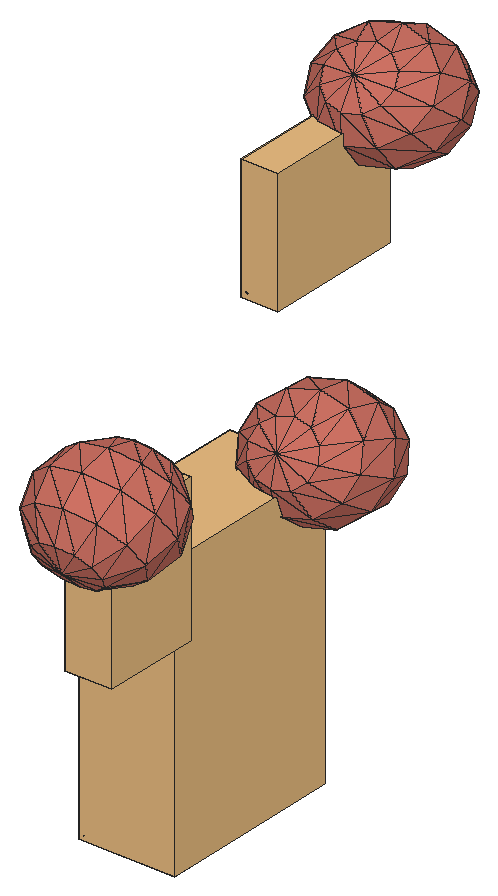
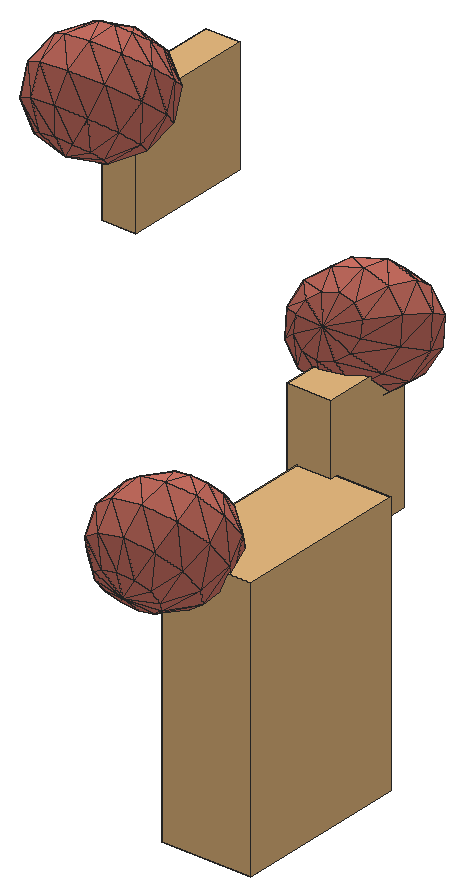
# SketchUp Ruby script. Lengths in inches.
U = 1.inch
M = Sketchup.active_model
def pt(a) = Geom::Point3d.new(a.map { |v| v * U })
def face(e, loops, mat)
  f = e.add_face(loops[0].map { |a| pt(a) })
  loops[1..].each { |l| e.add_face(l.map { |a| pt(a) }).erase! }
  f.material = f.back_material = mat if mat
  f
end
# faces: each face lists its corners as indices into pts; further lists are holes
def faces(e, pts, list, mat = nil) = list.each { |f| face(e, (f[0].is_a?(Array) ? f : [f]).map { |l| l.map { |i| pts[i] } }, mat) }
# xy, xz, yz: faces in a plane at the given z, y or x. An outline is a flat list of corners, or four numbers for a rectangle; further outlines are holes
def ring(l) = l.size == 4 ? [[l[0], l[1]], [l[2], l[1]], [l[2], l[3]], [l[0], l[3]]] : l.each_slice(2).to_a
def flat(e, list, mat, &to3) = list.each { |f| face(e, (f[0].is_a?(Array) ? f : [f]).map { |l| ring(l).map { |u, v| to3.(u, v) } }, mat) }
def xy(e, z, list, mat = nil) = flat(e, list, mat) { |x, y| [x, y, z] }
def xz(e, y, list, mat = nil) = flat(e, list, mat) { |x, z| [x, y, z] }
def yz(e, x, list, mat = nil) = flat(e, list, mat) { |y, z| [x, y, z] }
def lines(e, pts, list) = list.each { |a, b| e.add_line(pt(pts[a]), pt(pts[b])) }
# prism: a flat outline (further loops are holes) pulled along v
def prism(e, loops, v, mat = nil)
  f = face(e, loops, mat); d = Geom::Vector3d.new(v.map { |x| x * U })
  f.pushpull(f.normal.samedirection?(d) ? d.length : -d.length)
end
def box(e, o, s, mat = nil) = prism(e, [[o, [o[0] + s[0], o[1], o[2]], [o[0] + s[0], o[1] + s[1], o[2]], [o[0], o[1] + s[1], o[2]]]], [0, 0, s[2]], mat)
def at(x, y, z, deg = 0) = Geom::Transformation.translation(pt([x, y, z])) * Geom::Transformation.rotation(ORIGIN, Z_AXIS, deg.degrees)
def axes(o, x, y, z) = Geom::Transformation.new([*x, 0, *y, 0, *z, 0, *pt(o).to_a, 1])
def part(name) = M.definitions.add(name)
# library, detail: a bought-in or finely detailed component or shape, given as its bounding box
def library(name, o, s) = part(name).tap { |d| box(d.entities, o, s) }
def detail(e, o, s) = box(e.add_group.entities, o, s)
def put(e, d, t, mat = nil) = e.add_instance(d, t).tap { |i| i.material = mat if mat }
def group(e, t, mat = nil) = e.add_group.tap { |g| g.transformation = t; g.material = mat if mat }.entities
root = M.entities
M.materials.add("green").color = [174, 139, 102]
M.materials.add("vio").color = [206, 114, 100]
c1 = library("3DGeom~102_Defintion",[-331.46,-500,-168.38],[662.92,1000,336.76])
c2 = part("3DGeom~103_Defintion")
p = [[302.66,-500,-146.11],[317.99,-495.14,-154.33],[299.97,-497.07,-128.32],[317.99,-495.14,-154.33],[302.66,-500,-146.11],[309.56,-498.4,-152.34],
  [299.97,-497.07,-128.32],[317.99,-495.14,-154.33],[312.61,-489.29,-118.76],[312.61,-489.29,-118.76],[317.99,-495.14,-154.33],[327.95,-484.43,-126.98],
  [317.99,-495.14,-154.33],[325.71,-491.1,-151.56],[330.64,-487.36,-144.77],[327.95,-484.43,-126.98],[317.99,-495.14,-154.33],[330.64,-487.36,-144.77],
  [302.66,-500,-146.11],[299.97,-497.07,-128.32],[299.15,-499.51,-137.32],[327.95,-484.43,-126.98],[330.64,-487.36,-144.77],[331.46,-484.92,-135.77],
  [299.97,-497.07,-128.32],[312.61,-489.29,-118.76],[304.89,-493.33,-121.53],[312.61,-489.29,-118.76],[327.95,-484.43,-126.98],[321.05,-486.03,-120.75],
  [-317.36,495.99,133.65],[-331.46,484.07,150.24],[-328.26,482.74,159.03],[-317.36,495.99,133.65],[-328.26,482.74,159.03],[-321.59,483.72,165.67],
  [-317.36,495.99,133.65],[-321.59,483.72,165.67],[-313.24,486.75,168.38],[-317.36,495.99,133.65],[-330.32,487.36,141.66],[-331.46,484.07,150.24],
  [-317.36,495.99,133.65],[-313.24,486.75,168.38],[-305.4375,491.02,166.44],[-317.36,495.99,133.65],[-325.17,491.72,135.59],[-330.32,487.36,141.66],
  [-317.36,495.99,133.65],[-305.4375,491.02,166.44],[-300.28,495.38,160.37],[-317.36,495.99,133.65],[-300.28,495.38,160.37],[-299.15,498.67,151.79],
  [-317.36,495.99,133.65],[-299.15,498.67,151.79],[-302.34,500,143.01],[-317.36,495.99,133.65],[-302.34,500,143.01],[-309.01,499.02,136.36]]
faces(c2.entities,p,[[0,1,2],[3,4,5],[6,7,8],[9,10,11],[12,13,14],[15,16,17],[18,19,20],[21,22,23],
  [24,25,26],[27,28,29],[30,31,32],[33,34,35],[36,37,38],[39,40,41],[42,43,44],[45,46,47],
  [48,49,50],[51,52,53],[54,55,56],[57,58,59]],"green")
c3 = library("3DGeom~104_Defintion",[-334.52,-500,-160.51],[669.04,1000,321.02])
c4 = part("3DGeom~105_Defintion")
p = [[-306.36,-487.18,-90.84],[-301.3,-484.5,-160.51],[-278.52,-498.77,-106.98],[-278.52,-498.77,-106.98],[-301.3,-484.5,-160.51],[-275.99,-497.43,-141.8125],
  [-301.3,-484.5,-160.51],[-286.29,-491.76,-155.1],[-275.99,-497.43,-141.8125],[-331.67,-474.24,-109.53],[-301.3,-484.5,-160.51],[-306.36,-487.18,-90.84],
  [-329.14,-472.9,-144.36],[-301.3,-484.5,-160.51],[-331.67,-474.24,-109.53],[-301.3,-484.5,-160.51],[-329.14,-472.9,-144.36],[-316.98,-477.6,-156.58],
  [-329.14,-472.9,-144.36],[-331.67,-474.24,-109.53],[-334.52,-471.68,-127.14],[-278.52,-498.77,-106.98],[-275.99,-497.43,-141.8125],[-273.14,-500,-124.2],
  [-331.67,-474.24,-109.53],[-306.36,-487.18,-90.84],[-321.37,-479.92,-96.24],[-306.36,-487.18,-90.84],[-278.52,-498.77,-106.98],[-290.68,-494.08,-94.77],
  [313.125,494.74,102.45],[292.39,466.72,160.51],[309.13,461.51,157.36],[313.125,494.74,102.45],[309.13,461.51,157.36],[324.16,461.46,147.27],
  [313.125,494.74,102.45],[324.16,461.46,147.27],[333.45,466.57,132.95],[313.125,494.74,102.45],[333.45,466.57,132.95],[334.52,475.47,118.24],
  [313.125,494.74,102.45],[278.4375,475.68,155.88],[292.39,466.72,160.51],[313.125,494.74,102.45],[334.52,475.47,118.24],[327.08,485.78,107.08],
  [313.125,494.74,102.45],[271,485.99,144.72],[278.4375,475.68,155.88],[313.125,494.74,102.45],[272.07,494.89,130.01],[271,485.99,144.72],
  [313.125,494.74,102.45],[281.36,500,115.69],[272.07,494.89,130.01],[313.125,494.74,102.45],[296.39,499.94,105.61],[281.36,500,115.69]]
faces(c4.entities,p,[[0,1,2],[3,4,5],[6,7,8],[9,10,11],[12,13,14],[15,16,17],[18,19,20],[21,22,23],
  [24,25,26],[27,28,29],[30,31,32],[33,34,35],[36,37,38],[39,40,41],[42,43,44],[45,46,47],
  [48,49,50],[51,52,53],[54,55,56],[57,58,59]],"green")
c5 = part("3DGeom~222_Defintion")
p = [[138.17,-187.6,-427.375],[-199.9375,-99.75,-443.62],[24.02,0,-500],[340.4,-62.72,-359.51],[-304.37,62.72,-390.49],[340.4,-62.72,-359.51],
  [241.54,99.75,-422.41],[-96.57,187.6,-438.65],[-101.08,-262.21,-380.72],[-370.32,-172.76,-268.37],[-430.61,-78.97,-237.69],[-430.61,-78.97,-237.69],
  [-386.39,181.65,-235.57],[137.11,262.21,-369.28],[-386.39,181.65,-235.57],[-191.28,324.93,-259.77],[137.11,262.21,-369.28],[-191.28,324.93,-259.77],
  [215.3,-324.93,-240.23],[407.19,-181.65,-197.45],[407.19,-181.65,-197.45],[340.4,-62.72,-359.51],[451.41,78.97,-195.32],[340.4,-62.72,-359.51],
  [241.54,99.75,-422.41],[241.54,99.75,-422.41],[394.34,172.77,-231.63],[394.34,172.77,-231.63],[137.11,262.21,-369.28],[-304.37,62.72,-390.49],
  [-430.61,-78.97,-237.69],[-477.97,-10.3,-148.25],[-304.37,62.72,-390.49],[-386.39,181.65,-235.57],[-34.29,-381.14,-218.65],[-313.24,-266.5625,-232.06],
  [-101.08,-262.21,-380.72],[-34.29,-381.14,-218.65],[-313.24,-266.5625,-232.06],[394.34,172.77,-231.63],[137.11,262.21,-369.28],[334.05,266.5625,-200.96],
  [137.11,262.21,-369.28],[-191.28,324.93,-259.77],[55.09,381.14,-214.36],[334.05,266.5625,-200.96],[137.11,262.21,-369.28],[55.09,381.14,-214.36],
  [489.98,10.3,-101.75],[407.19,-181.65,-197.45],[-370.32,-172.76,-268.37],[-313.24,-266.5625,-232.06],[-441.48,-199.49,-21.21],[-370.32,-172.76,-268.37],
  [-191.28,324.93,-259.77],[-424.03,225.18,-20.37],[-191.28,324.93,-259.77],[-234.74,375.19,-11.28],[-191.28,324.93,-259.77],[-234.74,375.19,-11.28],
  [234.74,-375.19,11.28],[-34.29,-381.14,-218.65],[215.3,-324.93,-240.23],[424.03,-225.18,20.37],[234.74,-375.19,11.28],[215.3,-324.93,-240.23],
  [215.3,-324.93,-240.23],[-499.7,14.83,-24.01],[-34.29,-381.14,-218.65],[-274.68,-335.23,-138.48],[-313.24,-266.5625,-232.06],[-313.24,-266.5625,-232.06],
  [-274.68,-335.23,-138.48],[441.48,199.49,21.21],[334.05,266.5625,-200.96],[-17.45,-424.67,-0.84],[-34.29,-381.14,-218.65],[234.74,-375.19,11.28],
  [-34.29,-381.14,-218.65],[334.05,266.5625,-200.96],[286.69,335.23,-111.52],[286.69,335.23,-111.52],[17.45,424.67,0.84],[286.69,335.23,-111.52],
  [499.7,-14.83,24.01],[-264.96,-360.36,-12.73],[-274.68,-335.23,-138.48],[-264.96,-360.36,-12.73],[264.96,360.36,12.73],[286.69,335.23,-111.52],
  [264.96,360.36,12.73],[-489.98,-10.3,101.75],[-264.96,-360.36,-12.73],[-286.69,-335.23,111.52],[-286.69,-335.23,111.52],[-334.05,-266.5625,200.96],
  [-334.05,-266.5625,200.96],[-394.34,-172.77,231.63],[-451.41,-78.97,195.32],[-394.34,-172.77,231.63],[-407.19,181.65,197.45],[-234.74,375.19,-11.28],
  [-407.19,181.65,197.45],[-55.09,-381.14,214.36],[-286.69,-335.23,111.52],[-234.74,375.19,-11.28],[-407.19,181.65,197.45],[-215.3,324.93,240.23],
  [-215.3,324.93,240.23],[191.28,-324.93,259.77],[191.28,-324.93,259.77],[234.74,-375.19,11.28],[-215.3,324.93,240.23],[34.29,381.14,218.65],
  [264.96,360.36,12.73],[386.39,-181.65,235.57],[191.28,-324.93,259.77],[274.68,335.23,138.48],[264.96,360.36,12.73],[274.68,335.23,138.48],
  [477.97,10.3,148.25],[430.61,78.97,237.69],[370.32,172.77,268.37],[313.24,266.5625,232.06],[-407.19,181.65,197.45],[-137.11,-262.21,369.28],
  [-137.11,-262.21,369.28],[-334.05,-266.5625,200.96],[274.68,335.23,138.48],[101.08,262.21,380.72],[274.68,335.23,138.48],[101.08,262.21,380.72],
  [313.24,266.5625,232.06],[-340.4,62.72,359.51],[-394.34,-172.77,231.63],[-407.19,181.65,197.45],[-340.4,62.72,359.51],[-215.3,324.93,240.23],
  [-407.19,181.65,197.45],[-340.4,62.72,359.51],[-241.54,-99.75,422.41],[-394.34,-172.77,231.63],[-334.05,-266.5625,200.96],[-334.05,-266.5625,200.96],
  [-137.11,-262.21,369.28],[96.57,-187.6,438.65],[-55.09,-381.14,214.36],[-55.09,-381.14,214.36],[191.28,-324.93,259.77],[34.29,381.14,218.65],
  [-138.17,187.6,427.375],[34.29,381.14,218.65],[101.08,262.21,380.72],[-340.4,62.72,359.51],[-394.34,-172.77,231.63],[-241.54,-99.75,422.41],
  [313.24,266.5625,232.06],[199.9375,99.75,443.62],[313.24,266.5625,232.06],[370.32,172.77,268.37],[304.37,-62.72,390.49],[191.28,-324.93,259.77],
  [386.39,-181.65,235.57],[304.37,-62.72,390.49],[370.32,172.77,268.37],[304.37,-62.72,390.49],[430.61,78.97,237.69],[304.37,-62.72,390.49],
  [191.28,-324.93,259.77],[370.32,172.77,268.37],[304.37,-62.72,390.49],[-24.02,0,500],[304.37,-62.72,390.49]]
faces(c5.entities,p,[[0,1,2],[3,0,2],[2,1,4],[5,2,6],[2,4,7],[6,2,7],[8,9,1],[0,8,1],
  [1,9,10],[1,11,4],[7,4,12],[6,7,13],[7,14,15],[16,7,17],[18,8,0],[19,18,0],
  [20,0,21],[22,23,24],[22,25,26],[27,6,28],[29,30,31],[32,31,33],[34,35,36],[18,37,8],
  [8,38,9],[39,40,41],[42,43,44],[45,46,47],[48,49,23],[48,23,22],[50,51,52],[30,53,52],
  [54,33,55],[56,55,57],[47,58,59],[60,61,62],[63,64,65],[63,66,49],[31,30,52],[33,31,67],
  [33,67,55],[68,69,70],[71,72,52],[22,26,73],[26,74,73],[75,69,76],[77,75,78],[79,47,80],
  [81,47,82],[47,59,82],[74,83,73],[84,63,49],[84,49,48],[48,22,73],[67,31,52],[75,85,69],
  [86,87,52],[83,88,73],[89,82,90],[84,48,73],[91,67,52],[55,67,91],[92,93,52],[94,95,52],
  [96,97,52],[98,91,52],[99,98,52],[55,91,100],[101,55,102],[103,85,75],[103,104,85],[105,106,107],
  [82,59,108],[109,103,75],[110,75,111],[82,112,113],[114,82,113],[115,116,64],[115,64,63],[88,117,73],
  [118,113,119],[120,115,63],[120,63,84],[120,84,73],[121,120,73],[122,121,73],[123,122,73],[117,123,73],
  [124,91,98],[125,104,103],[126,127,104],[128,113,129],[130,131,132],[121,115,120],[133,98,134],[135,98,136],
  [137,138,139],[140,141,142],[140,143,144],[145,144,146],[145,147,148],[149,137,150],[151,150,152],[153,154,155],
  [156,152,157],[158,157,159],[160,161,162],[121,163,115],[164,165,166],[137,139,150],[167,145,168],[169,157,170],
  [150,139,140],[171,140,144],[171,144,145],[152,150,171],[152,171,157],[157,145,172],[150,140,171],[157,171,145]],"vio")
c6 = part("3DGeom~223_Defintion")
p = [[134.41,-263.08,-369.41],[-98.49,-186.72,-438.75],[24.02,0,-500],[240.51,-101.38,-422.46],[-198.9,101.38,-443.57],[240.51,-101.38,-422.46],
  [140.09,186.72,-427.28],[-98.38,263.08,-380.59],[-305,-60.32,-390.52],[-368.53,175.6,-268.28],[-310.49,268.95,-231.92],[-310.49,268.95,-231.92],
  [51.17,-381.46,-214.55],[-194.61,-323.41,-259.93],[51.17,-381.46,-214.55],[240.51,-101.38,-422.46],[341.03,60.32,-359.48],[341.03,60.32,-359.48],
  [218.625,323.41,-240.08],[-30.37,381.46,-218.47],[-30.37,381.46,-218.47],[218.625,323.41,-240.08],[331.3,-268.95,-201.09],[240.51,-101.38,-422.46],
  [331.3,-268.95,-201.09],[240.51,-101.38,-422.46],[392.55,-175.6,-231.72],[392.55,-175.6,-231.72],[240.51,-101.38,-422.46],[341.03,60.32,-359.48],
  [-388.24,-178.7,-235.66],[-388.24,-178.7,-235.66],[-429.78,82.24,-237.65],[-305,-60.32,-390.52],[-429.78,82.24,-237.65],[-98.38,263.08,-380.59],
  [-310.49,268.95,-231.92],[-271.23,337.3,-138.32],[-98.38,263.08,-380.59],[-30.37,381.46,-218.47],[283.24,-337.3,-111.68],[51.17,-381.46,-214.55],
  [134.41,-263.08,-369.41],[283.24,-337.3,-111.68],[134.41,-263.08,-369.41],[331.3,-268.95,-201.09],[450.59,-82.24,-195.36],[409.04,178.7,-197.36],
  [341.03,60.32,-359.48],[218.625,323.41,-240.08],[409.04,178.7,-197.36],[-368.53,175.6,-268.28],[-429.78,82.24,-237.65],[-439.41,202.76,-21.11],
  [-310.49,268.95,-231.92],[-368.53,175.6,-268.28],[13.09,-424.78,0.63],[-238.58,-373.4375,-11.46],[-194.61,-323.41,-259.93],[-194.61,-323.41,-259.93],
  [-238.58,-373.4375,-11.46],[-388.24,-178.7,-235.66],[-194.61,-323.41,-259.93],[218.625,323.41,-240.08],[238.58,373.4375,11.46],[218.625,323.41,-240.08],
  [-13.09,424.78,-0.63],[218.625,323.41,-240.08],[238.58,373.4375,11.46],[-388.24,-178.7,-235.66],[-477.84,13.89,-148.24],[-429.78,82.24,-237.65],
  [-429.78,82.24,-237.65],[-238.58,-373.4375,-11.46],[-426.32,-222.03,-20.48],[-388.24,-178.7,-235.66],[-388.24,-178.7,-235.66],[-271.23,337.3,-138.32],
  [-310.49,268.95,-231.92],[331.3,-268.95,-201.09],[439.41,-202.76,21.11],[-261.25,362.3125,-12.55],[261.25,-362.3125,12.55],[261.25,-362.3125,12.55],
  [283.24,-337.3,-111.68],[283.24,-337.3,-111.68],[489.85,-13.89,-101.76],[426.32,222.03,20.48],[-499.83,-11.125,-24.01],[-261.25,362.3125,-12.55],
  [-271.23,337.3,-138.32],[261.25,-362.3125,12.55],[499.83,11.125,24.01],[-409.04,-178.7,197.36],[-489.85,13.89,101.76],[-450.59,82.24,195.36],
  [-392.55,175.6,231.72],[-331.3,268.95,201.09],[-331.3,268.95,201.09],[-283.24,337.3,111.68],[-283.24,337.3,111.68],[-261.25,362.3125,-12.55],
  [-218.625,-323.41,240.08],[-238.58,-373.4375,-11.46],[-218.625,-323.41,240.08],[-283.24,337.3,111.68],[30.37,-381.46,218.47],[-218.625,-323.41,240.08],
  [-51.17,381.46,214.55],[238.58,373.4375,11.46],[-51.17,381.46,214.55],[271.23,-337.3,138.32],[271.23,-337.3,138.32],[261.25,-362.3125,12.55],
  [194.61,323.41,259.93],[238.58,373.4375,11.46],[-51.17,381.46,214.55],[194.61,323.41,259.93],[271.23,-337.3,138.32],[388.24,178.7,235.66],
  [194.61,323.41,259.93],[310.49,-268.95,231.92],[368.53,-175.6,268.28],[429.78,-82.24,237.65],[477.84,-13.89,148.24],[-341.03,-60.32,359.48],
  [-341.03,-60.32,359.48],[-51.17,381.46,214.55],[-331.3,268.95,201.09],[310.49,-268.95,231.92],[271.23,-337.3,138.32],[305,60.32,390.52],
  [305,60.32,390.52],[-240.51,101.38,422.46],[-341.03,-60.32,359.48],[-240.51,101.38,422.46],[-140.09,-186.72,427.28],[-409.04,-178.7,197.36],
  [-218.625,-323.41,240.08],[-341.03,-60.32,359.48],[-409.04,-178.7,197.36],[-134.41,263.08,369.41],[-331.3,268.95,201.09],[-392.55,175.6,231.72],
  [-51.17,381.46,214.55],[-331.3,268.95,201.09],[-134.41,263.08,369.41],[194.61,323.41,259.93],[-51.17,381.46,214.55],[98.38,-263.08,380.59],
  [-218.625,-323.41,240.08],[30.37,-381.46,218.47],[310.49,-268.95,231.92],[98.38,-263.08,380.59],[-392.55,175.6,231.72],[-240.51,101.38,422.46],
  [368.53,-175.6,268.28],[98.38,-263.08,380.59],[310.49,-268.95,231.92],[388.24,178.7,235.66],[98.49,186.72,438.74],[305,60.32,390.52],
  [388.24,178.7,235.66],[429.78,-82.24,237.65],[198.9,-101.38,443.57],[368.53,-175.6,268.28],[429.78,-82.24,237.65],[98.38,-263.08,380.59],
  [-218.625,-323.41,240.08],[368.53,-175.6,268.28],[98.38,-263.08,380.59],[-24.02,0,500],[98.38,-263.08,380.59]]
faces(c6.entities,p,[[0,1,2],[0,2,3],[1,4,2],[5,2,6],[2,4,7],[2,7,6],[1,8,4],[8,9,4],
  [4,9,10],[4,11,7],[12,13,1],[14,1,0],[13,8,1],[15,6,16],[17,6,18],[6,7,19],
  [6,20,21],[22,0,23],[24,25,26],[27,28,29],[13,30,8],[31,32,33],[8,34,9],[35,36,37],
  [38,37,39],[40,41,42],[43,44,45],[27,29,46],[46,29,47],[48,49,50],[51,52,53],[54,55,53],
  [56,57,58],[56,59,41],[60,61,62],[47,63,64],[65,39,66],[67,66,68],[69,70,71],[72,70,53],
  [73,74,75],[74,70,76],[77,78,53],[79,27,80],[27,46,80],[39,37,81],[39,81,66],[82,56,41],
  [83,41,84],[85,79,80],[46,47,86],[86,47,87],[47,64,87],[46,86,80],[74,88,70],[70,88,53],
  [89,90,53],[91,85,80],[86,92,80],[86,87,92],[93,88,74],[93,94,88],[88,94,53],[94,95,53],
  [95,96,53],[96,97,53],[98,99,53],[100,101,53],[102,74,103],[104,93,74],[66,81,105],[106,57,56],
  [106,107,57],[66,105,108],[109,66,110],[111,106,56],[112,56,113],[87,64,114],[115,116,117],[118,91,80],
  [92,87,119],[87,120,119],[121,118,80],[122,121,80],[123,122,80],[124,123,80],[92,124,80],[92,119,124],
  [125,94,93],[126,95,94],[127,105,128],[129,106,130],[124,131,123],[124,119,132],[133,95,134],[135,96,95],
  [136,137,138],[136,139,140],[141,142,143],[144,145,146],[147,148,141],[149,150,151],[152,153,106],[141,154,155],
  [156,157,158],[159,160,161],[162,147,160],[163,164,165],[166,161,164],[167,136,168],[147,141,160],[169,164,170],
  [171,139,136],[171,155,139],[160,141,155],[164,136,172],[161,171,164],[161,160,171],[160,155,171],[164,171,136]],"vio")
c7 = library("3DGeom~100_Defintion",[-500,-440.78,-130.77],[1000,881.57,261.54])
c8 = part("3DGeom~101_Defintion")
p = [[450.26,-438.5,-76.98],[473.93,-418.23,-130.77],[473.01,-420.54,-57.59],[450.72,-437.34,-113.57],[473.93,-418.23,-130.77],[450.26,-438.5,-76.98],
  [473.93,-418.23,-130.77],[450.72,-437.34,-113.57],[460.6,-429.08,-126.5],[473.01,-420.54,-57.59],[473.93,-418.23,-130.77],[496.21,-401.44,-74.78],
  [473.93,-418.23,-130.77],[487.14,-407.6875,-125.23],[496.68,-400.28,-111.37],[473.93,-418.23,-130.77],[496.68,-400.28,-111.37],[450.72,-437.34,-113.57],
  [450.26,-438.5,-76.98],[446.9375,-440.78,-95.45],[496.68,-400.28,-111.37],[500,-397.99,-92.9],[450.26,-438.5,-76.98],[473.01,-420.54,-57.59],
  [459.8,-431.09,-63.125],[473.01,-420.54,-57.59],[486.33,-409.69,-61.85],[-483.04,428.3125,67.76],[-497.53,394.8,97.99],[-487.96,391.61,113.91],
  [-483.04,428.3125,67.76],[-487.96,391.61,113.91],[-473.84,395.01,125.91],[-483.04,428.3125,67.76],[-500,403.73,82.41],[-497.53,394.8,97.99],
  [-483.04,428.3125,67.76],[-473.84,395.01,125.91],[-458.96,404.09,130.77],[-483.04,428.3125,67.76],[-494.7,415.99,71.34],[-483.04,428.3125,67.76],
  [-458.96,404.09,130.77],[-447.31,416.41,127.18],[-483.04,428.3125,67.76],[-447.31,416.41,127.18],[-442,428.67,116.12],[-483.04,428.3125,67.76],
  [-444.47,437.6,100.54],[-454.05,440.79,84.62],[-483.04,428.3125,67.76],[-454.05,440.79,84.62],[-468.16,437.39,72.62],[-483.04,428.3125,67.76],
  [-442,428.67,116.12],[-444.47,437.6,100.54]]
faces(c8.entities,p,[[0,1,2],[3,4,5],[6,7,8],[9,10,11],[12,13,14],[11,15,16],[17,18,19],[11,20,21],
  [22,23,24],[25,11,26],[27,28,29],[30,31,32],[33,34,35],[36,37,38],[39,40,34],[41,42,43],
  [44,45,46],[47,48,49],[50,51,52],[53,54,55]],"green")
c9 = part("3DGeom~221_Defintion")
p = [[192.89,-154.12,-424.75],[-160.54,-146.25,-441.73],[24.02,0,-500],[348.39,12.78,-359.13],[-312.36,-12.78,-390.87],[-151.29,154.12,-441.28],
  [202.15,146.25,-424.3],[348.39,12.78,-359.13],[-14.3,-279.72,-376.55],[-302.09,-253.31,-265.09],[-389.74,-176.26,-235.73],[-389.74,-176.26,-235.73],
  [-429.08,84.92,-237.62],[-429.08,84.92,-237.62],[-286.06,266.94,-264.32],[50.33,279.72,-373.45],[50.33,279.72,-373.45],[-286.06,266.94,-264.32],
  [310.08,-266.94,-235.68],[449.88,-84.92,-195.39],[310.08,-266.94,-235.68],[192.89,-154.12,-424.75],[192.89,-154.12,-424.75],[348.39,12.78,-359.13],
  [410.54,176.26,-197.28],[202.15,146.25,-424.3],[326.11,253.31,-234.91],[50.33,279.72,-373.45],[202.15,146.25,-424.3],[326.11,253.31,-234.91],
  [-312.36,-12.78,-390.87],[-389.74,-176.26,-235.73],[-457.125,-119.85,-147.25],[-312.36,-12.78,-390.87],[-429.08,84.92,-237.62],[87.19,-377.43,-212.82],
  [-217.65,-330.375,-227.46],[-14.3,-279.72,-376.55],[310.08,-266.94,-235.68],[87.19,-377.43,-212.82],[-217.65,-330.375,-227.46],[326.11,253.31,-234.91],
  [50.33,279.72,-373.45],[238.45,330.375,-205.55],[50.33,279.72,-373.45],[-286.06,266.94,-264.32],[-66.39,377.43,-220.19],[238.45,330.375,-205.55],
  [50.33,279.72,-373.45],[-66.39,377.43,-220.19],[469.14,119.85,-102.75],[-302.09,-253.31,-265.09],[-217.65,-330.375,-227.46],[-362.6875,-292.5,-17.42],
  [-302.09,-253.31,-265.09],[-362.6875,-292.5,-17.42],[-286.06,266.94,-264.32],[-479.41,120.6875,-23.03],[-286.06,266.94,-264.32],[-344.18,308.23,-16.53],
  [-286.06,266.94,-264.32],[-344.18,308.23,-16.53],[-486.1875,-99.2,-23.36],[344.18,-308.23,16.53],[87.19,-377.43,-212.82],[310.08,-266.94,-235.68],
  [479.41,-120.6875,23.03],[344.18,-308.23,16.53],[-362.6875,-292.5,-17.42],[362.6875,292.5,17.42],[238.45,330.375,-205.55],[-217.65,-330.375,-227.46],
  [-159.06,-386.79,-132.93],[-362.6875,-292.5,-17.42],[87.19,-377.43,-212.82],[-217.65,-330.375,-227.46],[-116.72,413.19,-5.61],[171.07,386.79,-117.07],
  [116.72,-413.19,5.61],[87.19,-377.43,-212.82],[344.18,-308.23,16.53],[87.19,-377.43,-212.82],[362.6875,292.5,17.42],[486.1875,99.2,23.36],
  [-362.6875,-292.5,-17.42],[-142.01,-407.43,-6.82],[142.01,407.43,6.82],[362.6875,292.5,17.42],[-469.14,-119.85,102.75],[-362.6875,-292.5,-17.42],
  [-449.88,84.92,195.39],[-344.18,308.23,-16.53],[-171.07,-386.79,117.07],[-238.45,-330.375,205.55],[-238.45,-330.375,205.55],[-326.11,-253.31,234.91],
  [-362.6875,-292.5,-17.42],[-410.54,-176.26,197.28],[-362.6875,-292.5,-17.42],[-326.11,-253.31,234.91],[-362.6875,-292.5,-17.42],[-344.18,308.23,-16.53],
  [-310.08,266.94,235.68],[-310.08,266.94,235.68],[66.39,-377.43,220.2],[-310.08,266.94,235.68],[-87.19,377.43,212.82],[286.06,-266.94,264.32],
  [286.06,-266.94,264.32],[344.18,-308.23,16.53],[159.06,386.79,132.93],[362.6875,292.5,17.42],[429.08,-84.92,237.62],[286.06,-266.94,264.32],
  [457.125,119.85,147.25],[389.74,176.26,235.73],[302.09,253.31,265.09],[217.65,330.375,227.46],[217.65,330.375,227.46],[362.6875,292.5,17.42],
  [-50.33,-279.72,373.45],[-50.33,-279.72,373.45],[14.3,279.72,376.55],[14.3,279.72,376.55],[217.65,330.375,227.46],[-348.39,-12.78,359.13],
  [-310.08,266.94,235.68],[-348.39,-12.78,359.13],[-348.39,-12.78,359.13],[-326.11,-253.31,234.91],[-202.15,-146.25,424.3],[-326.11,-253.31,234.91],
  [-238.45,-330.375,205.55],[-238.45,-330.375,205.55],[-50.33,-279.72,373.45],[-87.19,377.43,212.82],[-310.08,266.94,235.68],[-192.89,154.12,424.75],
  [-87.19,377.43,212.82],[14.3,279.72,376.55],[151.29,-154.12,441.28],[66.39,-377.43,220.2],[66.39,-377.43,220.2],[286.06,-266.94,264.32],
  [217.65,330.375,227.46],[160.54,146.25,441.73],[217.65,330.375,227.46],[302.09,253.31,265.09],[-348.39,-12.78,359.13],[-326.11,-253.31,234.91],
  [-202.15,-146.25,424.3],[312.36,12.78,390.87],[-310.08,266.94,235.68],[-348.39,-12.78,359.13],[-192.89,154.12,424.75],[302.09,253.31,265.09],
  [312.36,12.78,390.87],[389.74,176.26,235.73],[312.36,12.78,390.87],[286.06,-266.94,264.32],[429.08,-84.92,237.62],[312.36,12.78,390.87],
  [286.06,-266.94,264.32],[302.09,253.31,265.09],[312.36,12.78,390.87],[-348.39,-12.78,359.13],[-24.02,0,500],[312.36,12.78,390.87]]
faces(c9.entities,p,[[0,1,2],[3,0,2],[2,1,4],[2,4,5],[6,2,5],[7,2,6],[8,9,1],[0,8,1],
  [1,9,10],[1,11,4],[5,4,12],[5,13,14],[6,5,15],[16,5,17],[18,8,0],[19,20,21],
  [19,22,23],[24,23,25],[26,6,27],[24,28,29],[30,31,32],[33,32,34],[35,36,37],[38,39,8],
  [8,40,9],[41,42,43],[44,45,46],[47,48,49],[50,19,23],[50,23,24],[51,52,53],[31,54,55],
  [56,34,57],[58,57,59],[49,60,61],[34,32,62],[34,62,57],[63,64,65],[66,67,20],[32,31,68],
  [66,20,19],[24,29,69],[29,70,69],[71,72,73],[74,72,75],[49,61,76],[47,49,77],[77,49,76],
  [78,72,79],[80,78,81],[47,77,82],[50,24,69],[83,66,19],[83,19,50],[62,32,84],[78,85,72],
  [72,85,73],[77,86,87],[77,76,86],[83,50,69],[88,62,89],[57,62,88],[57,88,90],[91,57,90],
  [85,92,73],[92,93,73],[94,95,96],[97,88,98],[99,97,100],[101,90,102],[76,61,103],[104,85,78],
  [104,92,85],[76,105,106],[86,76,106],[107,104,78],[108,78,109],[86,110,111],[86,106,110],[112,113,67],
  [112,67,66],[114,83,69],[115,114,69],[116,115,69],[117,116,69],[110,118,119],[114,112,66],[114,66,83],
  [90,88,97],[120,93,92],[121,92,104],[110,106,122],[110,123,124],[115,112,114],[90,97,125],[126,90,127],
  [128,97,129],[130,131,132],[130,133,134],[135,136,137],[138,137,139],[140,134,141],[140,142,143],[144,139,145],
  [146,145,147],[148,149,150],[115,151,112],[152,153,154],[155,156,157],[158,159,160],[161,140,162],[163,145,164],
  [137,165,130],[166,130,134],[166,134,140],[139,137,166],[139,166,145],[145,140,167],[137,130,166],[145,166,140]],"vio")
g1 = group(root,at(15.3125,38.42,26.21))
put(g1,c1,axes([4,0.92,13.7],[0,0.00081,0],[0,0,-0.00081],[-0.00081,0,0]),"green")
put(g1,c2,axes([4,0.92,13.7],[0,0.00081,0],[0,0,-0.00081],[-0.00081,0,0]),"green")
g2 = group(root,at(15.3125,38.42,26.21))
put(g2,c3,axes([4.1,0.53,14.11],[0,0.00042,0],[0,0,-0.00042],[-0.00042,0,0]),"green")
put(g2,c4,axes([4.1,0.53,14.11],[0,0.00042,0],[0,0,-0.00042],[-0.00042,0,0]),"green")
g3 = group(root,at(15.3125,38.42,26.21))
put(g3,c5,axes([4.12,1.2,14.13],[0,0.00039,0],[0,0,-0.00039],[-0.00039,0,0]),"vio")
g4 = group(root,at(15.3125,38.42,26.21))
put(g4,c6,axes([4.16,0.38,14.35],[0,0.00039,0],[0,0,-0.00039],[-0.00039,0,0]),"vio")
g5 = group(root,at(15.3125,38.42,26.21))
put(g5,c7,axes([4.38,0.85,15.02],[0,0.0004,0],[0,0,-0.0004],[-0.0004,0,0]),"green")
put(g5,c8,axes([4.38,0.85,15.02],[0,0.0004,0],[0,0,-0.0004],[-0.0004,0,0]),"green")
g6 = group(root,at(15.3125,38.42,26.21))
put(g6,c9,axes([4.42,1.07,15.21],[0,0.00039,0],[0,0,-0.00039],[-0.00039,0,0]),"vio")
